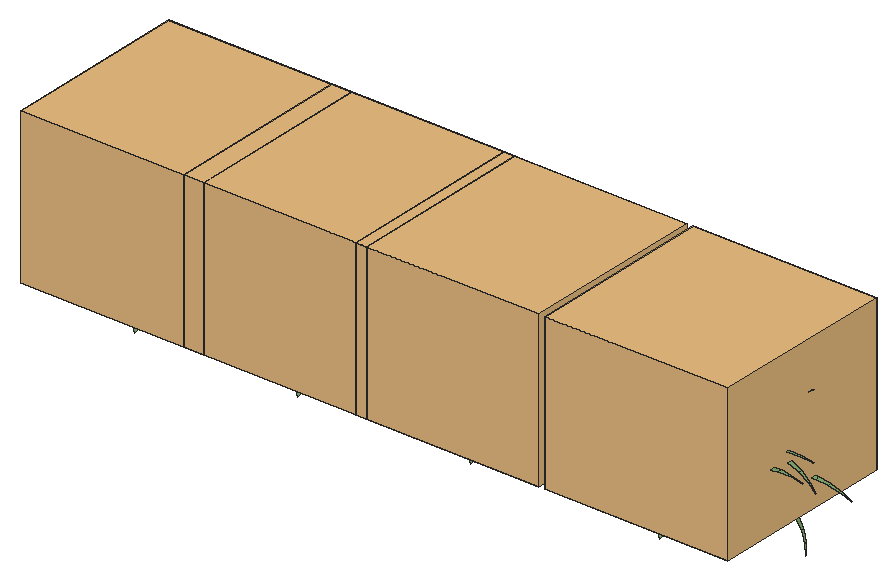
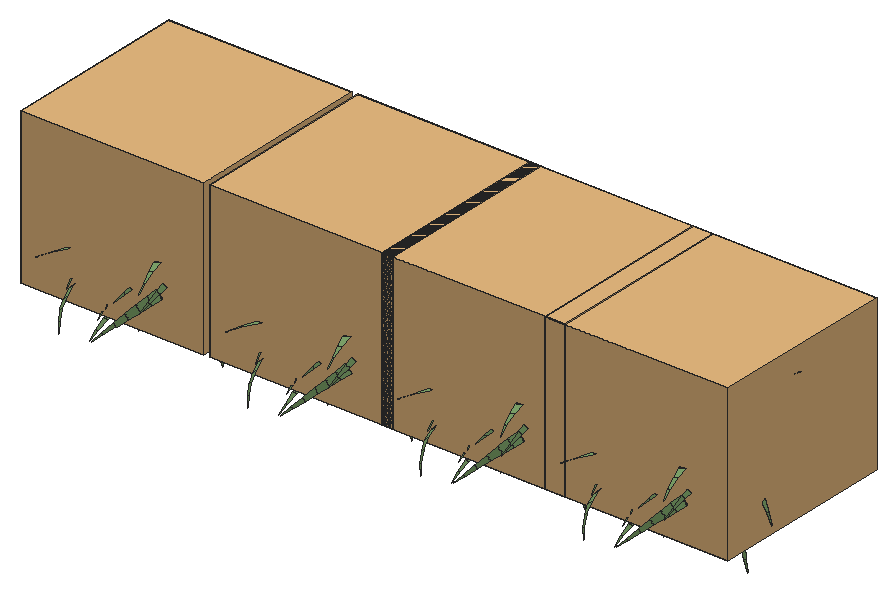
# SketchUp Ruby script. Lengths in inches.
U = 1.inch
M = Sketchup.active_model
def pt(a) = Geom::Point3d.new(a.map { |v| v * U })
def face(e, loops, mat)
  f = e.add_face(loops[0].map { |a| pt(a) })
  loops[1..].each { |l| e.add_face(l.map { |a| pt(a) }).erase! }
  f.material = f.back_material = mat if mat
  f
end
# faces: each face lists its corners as indices into pts; further lists are holes
def faces(e, pts, list, mat = nil) = list.each { |f| face(e, (f[0].is_a?(Array) ? f : [f]).map { |l| l.map { |i| pts[i] } }, mat) }
# xy, xz, yz: faces in a plane at the given z, y or x. An outline is a flat list of corners, or four numbers for a rectangle; further outlines are holes
def ring(l) = l.size == 4 ? [[l[0], l[1]], [l[2], l[1]], [l[2], l[3]], [l[0], l[3]]] : l.each_slice(2).to_a
def flat(e, list, mat, &to3) = list.each { |f| face(e, (f[0].is_a?(Array) ? f : [f]).map { |l| ring(l).map { |u, v| to3.(u, v) } }, mat) }
def xy(e, z, list, mat = nil) = flat(e, list, mat) { |x, y| [x, y, z] }
def xz(e, y, list, mat = nil) = flat(e, list, mat) { |x, z| [x, y, z] }
def yz(e, x, list, mat = nil) = flat(e, list, mat) { |y, z| [x, y, z] }
def lines(e, pts, list) = list.each { |a, b| e.add_line(pt(pts[a]), pt(pts[b])) }
# prism: a flat outline (further loops are holes) pulled along v
def prism(e, loops, v, mat = nil)
  f = face(e, loops, mat); d = Geom::Vector3d.new(v.map { |x| x * U })
  f.pushpull(f.normal.samedirection?(d) ? d.length : -d.length)
end
def box(e, o, s, mat = nil) = prism(e, [[o, [o[0] + s[0], o[1], o[2]], [o[0] + s[0], o[1] + s[1], o[2]], [o[0], o[1] + s[1], o[2]]]], [0, 0, s[2]], mat)
def at(x, y, z, deg = 0) = Geom::Transformation.translation(pt([x, y, z])) * Geom::Transformation.rotation(ORIGIN, Z_AXIS, deg.degrees)
def axes(o, x, y, z) = Geom::Transformation.new([*x, 0, *y, 0, *z, 0, *pt(o).to_a, 1])
def part(name) = M.definitions.add(name)
# library, detail: a bought-in or finely detailed component or shape, given as its bounding box
def library(name, o, s) = part(name).tap { |d| box(d.entities, o, s) }
def detail(e, o, s) = box(e.add_group.entities, o, s)
def put(e, d, t, mat = nil) = e.add_instance(d, t).tap { |i| i.material = mat if mat }
def group(e, t, mat = nil) = e.add_group.tap { |g| g.transformation = t; g.material = mat if mat }.entities
root = M.entities
M.materials.add("dianella").color = [131, 171, 111]
c1 = part("Shape Bender Component\#4")
p = [[0.27,1.78,0.46],[1.95,1.8,3.35],[1.95,4.67,3.35],[0.27,4.68,0.46],[3.06,1.81,4.8],[3.875,1.84,5.87],
  [3.875,4.64,5.87],[3.06,4.66,4.8],[6,1.9,8],[6,4.58,8],[27.35,3.23,6.09],[25.57,3.4375,7.9],
  [25.57,3.03,7.9],[23.28,2.8,9.61],[23.28,3.67,9.61],[7.08,1.93,8.8],[8.3,1.99,9.69],[8.3,4.5,9.69],
  [7.08,4.55,8.8],[23.04,2.78,9.74],[23.04,3.69,9.74],[20.86,3.86,10.86],[20.86,2.625,10.86],[10.73,2.08,10.92],
  [10.73,4.41,10.92],[12.13,2.13,11.33],[13.24,2.19,11.66],[13.24,4.3,11.66],[12.13,4.36,11.33],[18.35,2.46,11.63],
  [18.35,4.03,11.63],[15.79,2.32,11.89],[17.75,2.42,11.69],[17.75,4.07,11.69],[15.79,4.17,11.89]]
faces(c1.entities,p,[[0,1,2,3],[1,4,5,6,7,2],[5,8,9,6],[10,11,12],[13,12,11,14],[15,16,17,18,9,8],[19,13,14,20,21,22],[16,23,24,17],
  [23,25,26,27,28,24],[29,22,21,30],[31,32,29,30,33,34],[26,31,34,27]],"dianella")
c2 = part("Shape Bender Component\#7")
p = [[0.01,0.94,1.17],[0.04,0.96,6.32],[0.04,4.67,6.32],[0.01,4.68,1.17],[0.42,0.98,10.52],[0.51,1,11.45],
  [0.51,4.64,11.45],[0.42,4.66,10.52],[1.4,1.07,16.52],[1.4,4.57,16.52],[2.48,1.13,20.62],[2.71,1.16,21.49],
  [2.71,4.49,21.49],[2.48,4.52,20.625],[4.4375,1.21,26.32],[4.4375,4.46,26.32],[6.56,1.22,30.98],[6.56,4.47,30.98],
  [9.06,1.29,35.43],[9.06,4.38,35.43],[11.92,1.42,39.64],[11.92,4.23,39.64],[15.13,1.74,43.57],[15.13,4,43.57],
  [18.65,2.08,47.2],[18.65,3.67,47.2],[22.46,2.47,50.5],[22.46,3.14,50.5],[25.84,2.81,52.95]]
faces(c2.entities,p,[[0,1,2,3],[1,4,5,6,7,2],[5,8,9,6],[10,11,12,13,9,8],[11,14,15,12],[14,16,17,15],[16,18,19,17],[18,20,21,19],
  [20,22,23,21],[22,24,25,23],[24,26,27,25],[28,27,26]],"dianella")
c3 = part("Shape Bender Component\#5")
p = [[0.17,0.01,0.72],[1.09,0.03,4.5625],[1.09,3.73,4.5625],[0.17,3.75,0.72],[2.23,0.05,7.59],[2.48,0.0625,8.26],
  [2.48,3.71,8.26],[2.23,3.72,7.59],[4.33,0.14,11.74],[4.33,3.64,11.74],[6.2,0.2,14.41],[6.6,0.22,14.97],
  [6.6,3.56,14.97],[6.2,3.58,14.41],[9.26,0.35,17.88],[9.26,3.43,17.88],[12.27,0.4,20.43],[12.27,3.38,20.43],
  [15.58,0.51,22.59],[15.58,3.27,22.59],[19.13,0.73,24.3],[19.13,3.14,24.3],[22.875,1.08,25.56],[22.875,2.85,25.56],
  [26.75,1.47,26.33],[26.75,2.49,26.33],[30.68,1.86,26.6],[30.68,2.125,26.6],[33.95,1.875,26.45]]
faces(c3.entities,p,[[0,1,2,3],[1,4,5,6,7,2],[5,8,9,6],[8,10,11,12,13,9],[11,14,15,12],[14,16,17,15],[16,18,19,17],[18,20,21,19],
  [20,22,23,21],[22,24,25,23],[24,26,27,25],[28,27,26]],"dianella")
c4 = library("Trees & Plants  (59)",[-4.49,-4.79,-0.78],[10.02,10.13,10.22])
put(root,c1,axes([268.65,548.4,303.95],[-0.80569,0.56944,-0.02305],[0.57633,0.79454,-0.18542],[0.07749,0.17806,0.9833]))
put(root,c2,axes([270.24,546.25,295.18],[-0.89818,0.42386,0.09751],[0.36913,0.65726,0.03168],[0.04524,-0.03705,0.72823]))
put(root,c1,axes([266.02,544.48,305.64],[-0.51985,0.69677,-0.46908],[0.85127,0.46792,-0.24029],[-0.06489,0.54284,0.83687]))
put(root,c1,axes([268.17,544.76,295.79],[-0.45461,0.886,-0.06101],[0.85593,0.46132,0.22475],[-0.24461,-0.03601,0.9612]))
put(root,c1,axes([264.93,554.24,305.89],[-0.07554,0.99436,-0.05049],[0.89319,0.09828,0.42129],[-0.44228,0.02665,0.89336]))
put(root,c3,axes([270.08,550.61,299.04],[-0.33829,0.92096,-0.16447],[0.74479,0.29265,-0.04252],[-0.03806,0.18424,0.97431]))
put(root,c1,axes([265.76,560.98,305.84],[0.17955,0.96457,-0.21457],[0.72432,-0.00444,0.72223],[-0.65717,0.24154,0.6603]))
put(root,c1,axes([269.64,548.68,298.19],[-0.07554,0.99436,-0.05049],[0.89319,0.09828,0.42129],[-0.44228,0.02665,0.89336]))
put(root,c1,axes([266.85,552.72,301.24],[0.15821,0.98591,0.06027],[0.88231,-0.16242,0.42],[-0.44228,0.02665,0.89336]))
put(root,c4,axes([271.96,553.09,306.65],[4.356,0,0],[0,4.356,0],[0,0,3.6]))
put(root,c1,axes([268.55,551.76,296.11],[0.15821,0.98591,0.06027],[0.98524,-0.15399,-0.08295],[0.05813,-0.05813,0.98368]))
put(root,c1,axes([270.74,546.79,295.83],[0.26556,0.96121,-0.04549],[-0.85756,0.2684,0.37954],[0.43914,-0.059,0.80483]))
put(root,c1,axes([274.25,550.21,298.58],[0.03456,0.99793,0.05429],[-0.89708,0.01048,0.37838],[0.43914,-0.059,0.80483]))
put(root,c1,axes([278.54,553.69,293.96],[0.03456,0.99793,0.05429],[-0.99646,0.03857,-0.07473],[-0.06824,-0.04585,0.88619]))
put(root,c3,axes([269.89,548.07,296.59],[0.52067,0.83248,-0.14817],[-0.85026,0.52497,-0.03831],[0.06887,0.17559,0.87775]))
put(root,c1,axes([271.43,542.66,293.66],[0.61668,0.7819,-0.05497],[-0.7511,0.61748,0.20248],[0.2331,-0.08243,0.86594]))
put(root,c1,axes([276.92,558.11,302.72],[0.00951,0.98109,-0.1933],[-0.71163,0.13509,0.65066],[0.69138,0.1105,0.59486]))
put(root,c1,axes([276.44,551.34,302.77],[0.26556,0.96121,-0.04549],[-0.85756,0.2684,0.37954],[0.43914,-0.059,0.80483]))
put(root,c1,axes([270.83,546.12,299.32],[0.87579,0.38306,0.08831],[-0.40412,0.89443,-0.16738],[-0.06046,0.18068,0.91811]))
put(root,c2,axes([271.73,557.07,294.86],[0.94689,0.23499,0.20991],[0.15697,-0.72589,-0.13304],[-0.09792,-0.17134,0.70342]))
put(root,c1,axes([273.44,549.02,305.54],[0.82667,0.29857,0.38049],[-0.23842,0.92604,-0.27787],[-0.34507,0.20027,0.85088]))
put(root,c2,axes([272.14,553.52,294.52],[0.80902,-0.58527,0.05755],[-0.58572,-0.79585,0.15754],[0.03689,0.112,0.69708]))
put(root,c2,axes([275.85,548.43,293.12],[0.95837,0.27169,0.08785],[-0.27506,0.961,0.02854],[-0.05052,-0.03395,0.65606]))
put(root,c3,axes([269.61,552.34,294.5],[0.99357,-0.11272,0.01108],[-0.1132,-0.98932,0.09728],[0,0.08221,0.93937]))
put(root,c1,axes([272.32,547.65,304.22],[0.87743,-0.02048,-0.38891],[-0.15593,0.92511,-0.33346],[0.44545,0.37499,0.73497]))
put(root,c1,axes([275.33,552.81,306.52],[1,0,0],[0,-0.99572,0.09791],[0,0.08221,0.93937]))
put(root,c3,axes([274.08,549.94,293.42],[0.96956,-0.23675,0.0624],[0.23253,0.9702,0.0681],[-0.06824,-0.04585,0.88619]))
put(root,c1,axes([278.67,549.36,299.1],[0.95837,0.27169,0.08785],[-0.27506,0.961,0.02854],[-0.06824,-0.04585,0.88619]))
put(root,c3,axes([307.01,543.69,296.62],[-0.93269,0.35072,0.09345],[0.32759,0.91741,-0.21384],[0.14796,0.18564,0.96108]))
put(root,c1,axes([307.17,549.83,307.5],[-0.86496,0.14883,-0.43169],[0.33112,0.87778,-0.37014],[-0.36493,0.45373,0.81582]))
put(root,c3,axes([311.12,547.22,295.51],[-0.99701,-0.04566,0.06927],[-0.04139,0.99682,0.07559],[0.05813,-0.05813,0.98368]))
put(root,c1,axes([306.5,547.53,301.82],[-0.88813,0.45112,0.09751],[0.45492,0.89007,0.03168],[0.05813,-0.05813,0.98368]))
put(root,c1,axes([307.5625,548.4,303.95],[-0.80569,0.56944,-0.02305],[0.57633,0.79454,-0.18542],[0.07749,0.17806,0.9833]))
put(root,c2,axes([309.16,546.25,295.18],[-0.89818,0.42386,0.09751],[0.36913,0.65726,0.03168],[0.04524,-0.03705,0.72823]))
put(root,c1,axes([304.9375,544.48,305.64],[-0.51985,0.69677,-0.46908],[0.85127,0.46792,-0.24029],[-0.06489,0.54284,0.83687]))
put(root,c1,axes([307.08,544.76,295.79],[-0.45461,0.886,-0.06101],[0.85593,0.46132,0.22475],[-0.24461,-0.03601,0.9612]))
put(root,c1,axes([303.84,554.24,305.89],[-0.07554,0.99436,-0.05049],[0.89319,0.09828,0.42129],[-0.44228,0.02665,0.89336]))
put(root,c3,axes([308.99,550.61,299.04],[-0.33829,0.92096,-0.16447],[0.74479,0.29265,-0.04252],[-0.03806,0.18424,0.97431]))
put(root,c1,axes([304.67,560.98,305.84],[0.17955,0.96457,-0.21457],[0.72432,-0.00444,0.72223],[-0.65717,0.24154,0.6603]))
put(root,c1,axes([308.56,548.68,298.19],[-0.07554,0.99436,-0.05049],[0.89319,0.09828,0.42129],[-0.44228,0.02665,0.89336]))
put(root,c1,axes([305.77,552.72,301.24],[0.15821,0.98591,0.06027],[0.88231,-0.16242,0.42],[-0.44228,0.02665,0.89336]))
put(root,c4,axes([310.87,553.09,306.65],[4.356,0,0],[0,4.356,0],[0,0,3.6]))
put(root,c1,axes([307.47,551.76,296.11],[0.15821,0.98591,0.06027],[0.98524,-0.15399,-0.08295],[0.05813,-0.05813,0.98368]))
put(root,c1,axes([309.65,546.79,295.83],[0.26556,0.96121,-0.04549],[-0.85756,0.2684,0.37954],[0.43914,-0.059,0.80483]))
put(root,c1,axes([313.17,550.21,298.58],[0.03456,0.99793,0.05429],[-0.89708,0.01048,0.37838],[0.43914,-0.059,0.80483]))
put(root,c1,axes([317.46,553.69,293.96],[0.03456,0.99793,0.05429],[-0.99646,0.03857,-0.07473],[-0.06824,-0.04585,0.88619]))
put(root,c3,axes([308.8,548.07,296.59],[0.52067,0.83248,-0.14817],[-0.85026,0.52497,-0.03831],[0.06887,0.17559,0.87775]))
put(root,c1,axes([310.34,542.66,293.66],[0.61668,0.7819,-0.05497],[-0.7511,0.61748,0.20248],[0.2331,-0.08243,0.86594]))
put(root,c1,axes([315.83,558.11,302.72],[0.00951,0.98109,-0.1933],[-0.71163,0.13509,0.65066],[0.69138,0.1105,0.59486]))
put(root,c1,axes([315.35,551.34,302.77],[0.26556,0.96121,-0.04549],[-0.85756,0.2684,0.37954],[0.43914,-0.059,0.80483]))
put(root,c1,axes([309.75,546.12,299.32],[0.87579,0.38306,0.08831],[-0.40412,0.89443,-0.16738],[-0.06046,0.18068,0.91811]))
put(root,c2,axes([310.65,557.07,294.86],[0.94689,0.23499,0.20991],[0.15697,-0.72589,-0.13304],[-0.09792,-0.17134,0.70342]))
put(root,c1,axes([312.35,549.02,305.54],[0.82667,0.29857,0.38049],[-0.23842,0.92604,-0.27787],[-0.34507,0.20027,0.85088]))
put(root,c2,axes([311.06,553.52,294.52],[0.80902,-0.58527,0.05755],[-0.58572,-0.79585,0.15754],[0.03689,0.112,0.69708]))
put(root,c2,axes([314.77,548.43,293.12],[0.95837,0.27169,0.08785],[-0.27506,0.961,0.02854],[-0.05052,-0.03395,0.65606]))
put(root,c3,axes([308.52,552.34,294.5],[0.99357,-0.11272,0.01108],[-0.1132,-0.98932,0.09728],[0,0.08221,0.93937]))
put(root,c1,axes([311.24,547.65,304.22],[0.87743,-0.02048,-0.38891],[-0.15593,0.92511,-0.33346],[0.44545,0.37499,0.73497]))
put(root,c1,axes([314.25,552.81,306.52],[1,0,0],[0,-0.99572,0.09791],[0,0.08221,0.93937]))
put(root,c3,axes([313,549.94,293.42],[0.96956,-0.23675,0.0624],[0.23253,0.9702,0.0681],[-0.06824,-0.04585,0.88619]))
put(root,c1,axes([317.59,549.36,299.1],[0.95837,0.27169,0.08785],[-0.27506,0.961,0.02854],[-0.06824,-0.04585,0.88619]))
put(root,c1,axes([347.08,544.77,301.91],[-0.98591,-0.15821,0.06027],[-0.15399,0.98524,0.08295],[0.05813,-0.05813,0.98368]))
put(root,c3,axes([348.1,543.69,296.62],[-0.93269,0.35072,0.09345],[0.32759,0.91741,-0.21384],[0.14796,0.18564,0.96108]))
put(root,c1,axes([348.26,549.83,307.5],[-0.86496,0.14883,-0.43169],[0.33112,0.87778,-0.37014],[-0.36493,0.45373,0.81582]))
put(root,c3,axes([352.21,547.22,295.51],[-0.99701,-0.04566,0.06927],[-0.04139,0.99682,0.07559],[0.05813,-0.05813,0.98368]))
put(root,c1,axes([347.6,547.53,301.82],[-0.88813,0.45112,0.09751],[0.45492,0.89007,0.03168],[0.05813,-0.05813,0.98368]))
put(root,c1,axes([348.66,548.4,303.95],[-0.80569,0.56944,-0.02305],[0.57633,0.79454,-0.18542],[0.07749,0.17806,0.9833]))
put(root,c2,axes([350.25,546.25,295.18],[-0.89818,0.42386,0.09751],[0.36913,0.65726,0.03168],[0.04524,-0.03705,0.72823]))
put(root,c1,axes([346.03,544.48,305.64],[-0.51985,0.69677,-0.46908],[0.85127,0.46792,-0.24029],[-0.06489,0.54284,0.83687]))
put(root,c1,axes([348.18,544.76,295.79],[-0.45461,0.886,-0.06101],[0.85593,0.46132,0.22475],[-0.24461,-0.03601,0.9612]))
put(root,c1,axes([344.94,554.24,305.89],[-0.07554,0.99436,-0.05049],[0.89319,0.09828,0.42129],[-0.44228,0.02665,0.89336]))
put(root,c3,axes([350.09,550.61,299.04],[-0.33829,0.92096,-0.16447],[0.74479,0.29265,-0.04252],[-0.03806,0.18424,0.97431]))
put(root,c1,axes([345.77,560.98,305.84],[0.17955,0.96457,-0.21457],[0.72432,-0.00444,0.72223],[-0.65717,0.24154,0.6603]))
put(root,c1,axes([349.65,548.68,298.19],[-0.07554,0.99436,-0.05049],[0.89319,0.09828,0.42129],[-0.44228,0.02665,0.89336]))
put(root,c1,axes([346.86,552.72,301.24],[0.15821,0.98591,0.06027],[0.88231,-0.16242,0.42],[-0.44228,0.02665,0.89336]))
put(root,c4,axes([351.97,553.09,306.65],[4.356,0,0],[0,4.356,0],[0,0,3.6]))
put(root,c1,axes([348.5625,551.76,296.11],[0.15821,0.98591,0.06027],[0.98524,-0.15399,-0.08295],[0.05813,-0.05813,0.98368]))
put(root,c1,axes([350.75,546.79,295.83],[0.26556,0.96121,-0.04549],[-0.85756,0.2684,0.37954],[0.43914,-0.059,0.80483]))
put(root,c1,axes([354.26,550.21,298.58],[0.03456,0.99793,0.05429],[-0.89708,0.01048,0.37838],[0.43914,-0.059,0.80483]))
put(root,c1,axes([358.55,553.69,293.96],[0.03456,0.99793,0.05429],[-0.99646,0.03857,-0.07473],[-0.06824,-0.04585,0.88619]))
put(root,c3,axes([349.9,548.07,296.59],[0.52067,0.83248,-0.14817],[-0.85026,0.52497,-0.03831],[0.06887,0.17559,0.87775]))
put(root,c1,axes([351.4375,542.66,293.66],[0.61668,0.7819,-0.05497],[-0.7511,0.61748,0.20248],[0.2331,-0.08243,0.86594]))
put(root,c1,axes([356.93,558.11,302.72],[0.00951,0.98109,-0.1933],[-0.71163,0.13509,0.65066],[0.69138,0.1105,0.59486]))
put(root,c1,axes([356.45,551.34,302.77],[0.26556,0.96121,-0.04549],[-0.85756,0.2684,0.37954],[0.43914,-0.059,0.80483]))
put(root,c1,axes([350.84,546.12,299.32],[0.87579,0.38306,0.08831],[-0.40412,0.89443,-0.16738],[-0.06046,0.18068,0.91811]))
put(root,c2,axes([351.74,557.07,294.86],[0.94689,0.23499,0.20991],[0.15697,-0.72589,-0.13304],[-0.09792,-0.17134,0.70342]))
put(root,c1,axes([353.45,549.02,305.54],[0.82667,0.29857,0.38049],[-0.23842,0.92604,-0.27787],[-0.34507,0.20027,0.85088]))
put(root,c2,axes([352.15,553.52,294.52],[0.80902,-0.58527,0.05755],[-0.58572,-0.79585,0.15754],[0.03689,0.112,0.69708]))
put(root,c2,axes([355.86,548.43,293.12],[0.95837,0.27169,0.08785],[-0.27506,0.961,0.02854],[-0.05052,-0.03395,0.65606]))
put(root,c3,axes([349.62,552.34,294.5],[0.99357,-0.11272,0.01108],[-0.1132,-0.98932,0.09728],[0,0.08221,0.93937]))
put(root,c1,axes([352.33,547.65,304.22],[0.87743,-0.02048,-0.38891],[-0.15593,0.92511,-0.33346],[0.44545,0.37499,0.73497]))
put(root,c1,axes([355.34,552.81,306.52],[1,0,0],[0,-0.99572,0.09791],[0,0.08221,0.93937]))
put(root,c3,axes([354.09,549.94,293.42],[0.96956,-0.23675,0.0624],[0.23253,0.9702,0.0681],[-0.06824,-0.04585,0.88619]))
put(root,c1,axes([358.68,549.36,299.1],[0.95837,0.27169,0.08785],[-0.27506,0.961,0.02854],[-0.06824,-0.04585,0.88619]))
put(root,c3,axes([393.21,543.69,296.62],[-0.93269,0.35072,0.09345],[0.32759,0.91741,-0.21384],[0.14796,0.18564,0.96108]))
put(root,c1,axes([393.37,549.83,307.5],[-0.86496,0.14883,-0.43169],[0.33112,0.87778,-0.37014],[-0.36493,0.45373,0.81582]))
put(root,c3,axes([397.32,547.22,295.51],[-0.99701,-0.04566,0.06927],[-0.04139,0.99682,0.07559],[0.05813,-0.05813,0.98368]))
put(root,c1,axes([392.71,547.53,301.82],[-0.88813,0.45112,0.09751],[0.45492,0.89007,0.03168],[0.05813,-0.05813,0.98368]))
put(root,c1,axes([393.77,548.4,303.95],[-0.80569,0.56944,-0.02305],[0.57633,0.79454,-0.18542],[0.07749,0.17806,0.9833]))
put(root,c2,axes([395.36,546.25,295.18],[-0.89818,0.42386,0.09751],[0.36913,0.65726,0.03168],[0.04524,-0.03705,0.72823]))
put(root,c1,axes([391.14,544.48,305.64],[-0.51985,0.69677,-0.46908],[0.85127,0.46792,-0.24029],[-0.06489,0.54284,0.83687]))
put(root,c1,axes([393.29,544.76,295.79],[-0.45461,0.886,-0.06101],[0.85593,0.46132,0.22475],[-0.24461,-0.03601,0.9612]))
put(root,c1,axes([390.05,554.24,305.89],[-0.07554,0.99436,-0.05049],[0.89319,0.09828,0.42129],[-0.44228,0.02665,0.89336]))
put(root,c3,axes([395.2,550.61,299.04],[-0.33829,0.92096,-0.16447],[0.74479,0.29265,-0.04252],[-0.03806,0.18424,0.97431]))
put(root,c1,axes([390.88,560.98,305.84],[0.17955,0.96457,-0.21457],[0.72432,-0.00444,0.72223],[-0.65717,0.24154,0.6603]))
put(root,c1,axes([394.76,548.68,298.19],[-0.07554,0.99436,-0.05049],[0.89319,0.09828,0.42129],[-0.44228,0.02665,0.89336]))
put(root,c1,axes([391.97,552.72,301.24],[0.15821,0.98591,0.06027],[0.88231,-0.16242,0.42],[-0.44228,0.02665,0.89336]))
put(root,c4,axes([397.08,553.09,306.65],[4.356,0,0],[0,4.356,0],[0,0,3.6]))
put(root,c1,axes([393.67,551.76,296.11],[0.15821,0.98591,0.06027],[0.98524,-0.15399,-0.08295],[0.05813,-0.05813,0.98368]))
put(root,c1,axes([395.86,546.79,295.83],[0.26556,0.96121,-0.04549],[-0.85756,0.2684,0.37954],[0.43914,-0.059,0.80483]))
put(root,c1,axes([399.37,550.21,298.58],[0.03456,0.99793,0.05429],[-0.89708,0.01048,0.37838],[0.43914,-0.059,0.80483]))
put(root,c1,axes([403.66,553.69,293.96],[0.03456,0.99793,0.05429],[-0.99646,0.03857,-0.07473],[-0.06824,-0.04585,0.88619]))
put(root,c3,axes([395.01,548.07,296.59],[0.52067,0.83248,-0.14817],[-0.85026,0.52497,-0.03831],[0.06887,0.17559,0.87775]))
put(root,c1,axes([396.55,542.66,293.66],[0.61668,0.7819,-0.05497],[-0.7511,0.61748,0.20248],[0.2331,-0.08243,0.86594]))
put(root,c1,axes([402.04,558.11,302.72],[0.00951,0.98109,-0.1933],[-0.71163,0.13509,0.65066],[0.69138,0.1105,0.59486]))
put(root,c1,axes([401.56,551.34,302.77],[0.26556,0.96121,-0.04549],[-0.85756,0.2684,0.37954],[0.43914,-0.059,0.80483]))
put(root,c1,axes([395.95,546.12,299.32],[0.87579,0.38306,0.08831],[-0.40412,0.89443,-0.16738],[-0.06046,0.18068,0.91811]))
put(root,c2,axes([396.85,557.07,294.86],[0.94689,0.23499,0.20991],[0.15697,-0.72589,-0.13304],[-0.09792,-0.17134,0.70342]))
put(root,c1,axes([398.56,549.02,305.54],[0.82667,0.29857,0.38049],[-0.23842,0.92604,-0.27787],[-0.34507,0.20027,0.85088]))
put(root,c2,axes([397.26,553.52,294.52],[0.80902,-0.58527,0.05755],[-0.58572,-0.79585,0.15754],[0.03689,0.112,0.69708]))
put(root,c2,axes([400.97,548.43,293.12],[0.95837,0.27169,0.08785],[-0.27506,0.961,0.02854],[-0.05052,-0.03395,0.65606]))
put(root,c3,axes([394.73,552.34,294.5],[0.99357,-0.11272,0.01108],[-0.1132,-0.98932,0.09728],[0,0.08221,0.93937]))
put(root,c1,axes([397.44,547.65,304.22],[0.87743,-0.02048,-0.38891],[-0.15593,0.92511,-0.33346],[0.44545,0.37499,0.73497]))
put(root,c1,axes([400.45,552.81,306.52],[1,0,0],[0,-0.99572,0.09791],[0,0.08221,0.93937]))
put(root,c3,axes([399.2,549.94,293.42],[0.96956,-0.23675,0.0624],[0.23253,0.9702,0.0681],[-0.06824,-0.04585,0.88619]))
put(root,c1,axes([403.79,549.36,299.1],[0.95837,0.27169,0.08785],[-0.27506,0.961,0.02854],[-0.06824,-0.04585,0.88619]))
